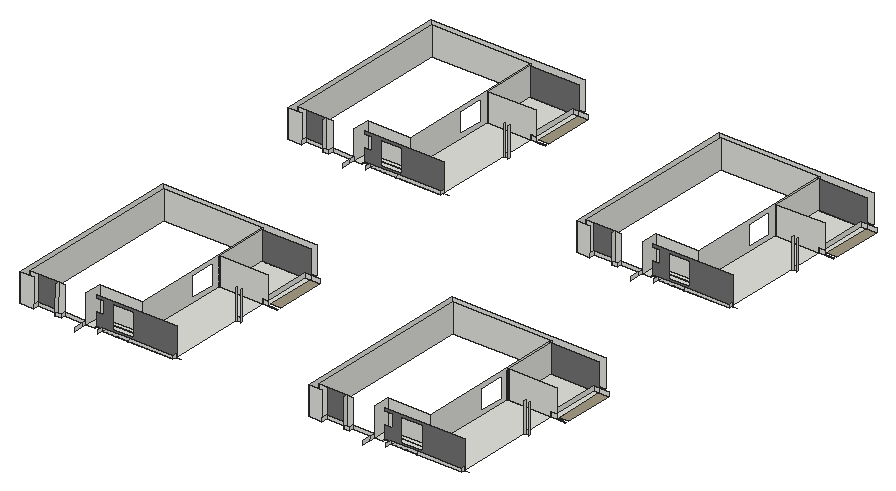
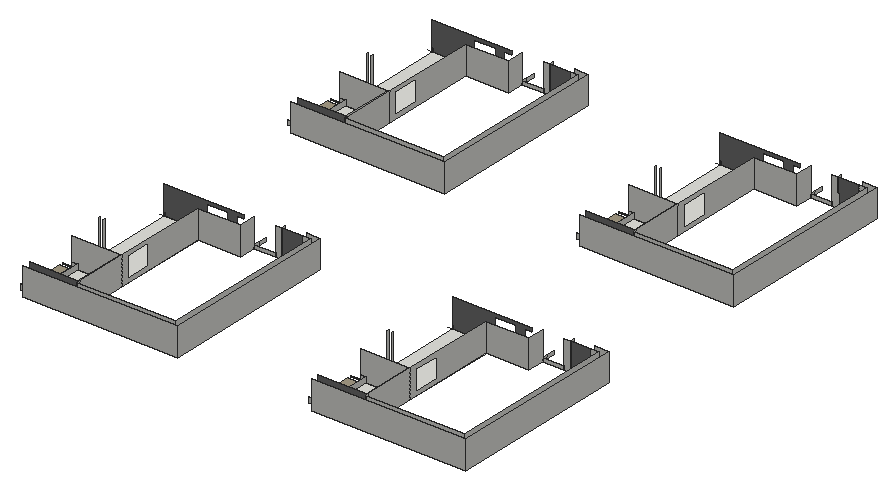
# SketchUp Ruby script. Lengths in inches.
U = 1.inch
M = Sketchup.active_model
def pt(a) = Geom::Point3d.new(a.map { |v| v * U })
def face(e, loops, mat)
  f = e.add_face(loops[0].map { |a| pt(a) })
  loops[1..].each { |l| e.add_face(l.map { |a| pt(a) }).erase! }
  f.material = f.back_material = mat if mat
  f
end
# faces: each face lists its corners as indices into pts; further lists are holes
def faces(e, pts, list, mat = nil) = list.each { |f| face(e, (f[0].is_a?(Array) ? f : [f]).map { |l| l.map { |i| pts[i] } }, mat) }
# xy, xz, yz: faces in a plane at the given z, y or x. An outline is a flat list of corners, or four numbers for a rectangle; further outlines are holes
def ring(l) = l.size == 4 ? [[l[0], l[1]], [l[2], l[1]], [l[2], l[3]], [l[0], l[3]]] : l.each_slice(2).to_a
def flat(e, list, mat, &to3) = list.each { |f| face(e, (f[0].is_a?(Array) ? f : [f]).map { |l| ring(l).map { |u, v| to3.(u, v) } }, mat) }
def xy(e, z, list, mat = nil) = flat(e, list, mat) { |x, y| [x, y, z] }
def xz(e, y, list, mat = nil) = flat(e, list, mat) { |x, z| [x, y, z] }
def yz(e, x, list, mat = nil) = flat(e, list, mat) { |y, z| [x, y, z] }
def lines(e, pts, list) = list.each { |a, b| e.add_line(pt(pts[a]), pt(pts[b])) }
# prism: a flat outline (further loops are holes) pulled along v
def prism(e, loops, v, mat = nil)
  f = face(e, loops, mat); d = Geom::Vector3d.new(v.map { |x| x * U })
  f.pushpull(f.normal.samedirection?(d) ? d.length : -d.length)
end
def box(e, o, s, mat = nil) = prism(e, [[o, [o[0] + s[0], o[1], o[2]], [o[0] + s[0], o[1] + s[1], o[2]], [o[0], o[1] + s[1], o[2]]]], [0, 0, s[2]], mat)
def at(x, y, z, deg = 0) = Geom::Transformation.translation(pt([x, y, z])) * Geom::Transformation.rotation(ORIGIN, Z_AXIS, deg.degrees)
def axes(o, x, y, z) = Geom::Transformation.new([*x, 0, *y, 0, *z, 0, *pt(o).to_a, 1])
def part(name) = M.definitions.add(name)
# library, detail: a bought-in or finely detailed component or shape, given as its bounding box
def library(name, o, s) = part(name).tap { |d| box(d.entities, o, s) }
def detail(e, o, s) = box(e.add_group.entities, o, s)
def put(e, d, t, mat = nil) = e.add_instance(d, t).tap { |i| i.material = mat if mat }
def group(e, t, mat = nil) = e.add_group.tap { |g| g.transformation = t; g.material = mat if mat }.entities
root = M.entities
M.materials.add("[Color M05]").color = [114, 114, 114]
M.materials.add("[Concrete Tile]").color = [165, 155, 133]
M.materials.add("[Granite Brown]").color = [89, 59, 61]
xy(root,1264.5625,[[653.67,1822.9375,653.67,1835.1875,557.4,1835.1875,557.4,1875.8125,704.25,1875.8125,704.25,1822.9375],[1871.86,1822.9375,1871.86,1835.1875,1775.59,1835.1875,1775.59,1875.8125,1922.4375,1875.8125,1922.4375,1822.9375],[557.4,1833.3125,653.67,1835.1875],[1775.59,1833.3125,1871.86,1835.1875],[653.67,3237.625,653.67,3249.875,557.4,3249.875,557.4,3290.5,704.25,3290.5,704.25,3237.625],
  [1871.86,3237.625,1871.86,3249.875,1775.59,3249.875,1775.59,3290.5,1922.4375,3290.5,1922.4375,3237.625],[557.4,3248,653.67,3249.875],[1775.59,3248,1871.86,3249.875]])
xy(root,1264.6875,[[653.67,1822.9375,704.25,1822.9375,704.25,1835.1875,557.4,1835.1875,557.4,1833.3125,653.67,1833.3125],[1871.86,1822.9375,1922.4375,1822.9375,1922.4375,1835.1875,1775.59,1835.1875,1775.59,1833.3125,1871.86,1833.3125],[653.67,3237.625,704.25,3237.625,704.25,3249.875,557.4,3249.875,557.4,3248,653.67,3248],[1871.86,3237.625,1922.4375,3237.625,1922.4375,3249.875,1775.59,3249.875,1775.59,3248,1871.86,3248]])
xy(root,1266,[[523.04,1822.9375,557.4,1893.6875],[704.25,1822.9375,890.875,1835.1875],[1741.23,1822.9375,1775.59,1893.6875],[1922.4375,1822.9375,2109.0625,1835.1875],[557.4,1835.1875,704.25,1875.8125],
  [704.25,1835.1875,890.875,2295.875],[1775.59,1835.1875,1922.4375,1875.8125],[1922.4375,1835.1875,2109.0625,2295.875],[557.4,1875.8125,704.25,1893.6875],[1775.59,1875.8125,1922.4375,1893.6875],
  [704.25,2295.875,710.125,2518.89],[710.125,2295.875,890.875,2518.89],[890.875,2295.875,913.875,2518.89],[1922.4375,2295.875,1928.3125,2518.89],[1928.3125,2295.875,2109.0625,2518.89],
  [2109.0625,2295.875,2132.0625,2518.89],[704.25,2518.89,890.875,2531.375],[1922.4375,2518.89,2109.0625,2531.375],[523.04,3237.625,557.4,3308.375],[704.25,3237.625,890.875,3249.875],
  [1741.23,3237.625,1775.59,3308.375],[1922.4375,3237.625,2109.0625,3249.875],[557.4,3249.875,704.25,3290.5],[704.25,3249.875,890.875,3710.5625],[1775.59,3249.875,1922.4375,3290.5],
  [1922.4375,3249.875,2109.0625,3710.5625],[557.4,3290.5,704.25,3308.375],[1775.59,3290.5,1922.4375,3308.375],[704.25,3710.5625,710.125,3933.57],[710.125,3710.5625,890.875,3933.57],
  [890.875,3710.5625,913.875,3933.57],[1922.4375,3710.5625,1928.3125,3933.57],[1928.3125,3710.5625,2109.0625,3933.57],[2109.0625,3710.5625,2132.0625,3933.57],[704.25,3933.57,890.875,3946.0625],
  [1922.4375,3933.57,2109.0625,3946.0625]])
xy(root,1266,[[913.875,2310.68,954.6875,2518.89],[2132.0625,2310.68,2172.875,2518.89],[913.875,3725.37,954.6875,3933.57],[2132.0625,3725.37,2172.875,3933.57]],"[Concrete Tile]")
xy(root,1266,[[557.4,1822.9375,557.88,1833.3125],[1775.59,1822.9375,1776.07,1833.3125],[557.4,1833.3125,557.88,1835.1875],[1775.59,1833.3125,1776.07,1835.1875],[557.4,3237.625,557.88,3248],
  [1775.59,3237.625,1776.07,3248],[557.4,3248,557.88,3249.875],[1775.59,3248,1776.07,3249.875]],"[Granite Brown]")
xz(root,1799.9375,[[262.875,1266,319.53,1386],[1481.0625,1266,1537.72,1386]])
xz(root,1806.5625,[[404.95,1266,404.95,1281.4375,405.03,1281.4375],[404.95,1266,431.33,1266,431.33,1281.4375,405.03,1281.4375],[1623.14,1266,1623.14,1281.4375,1623.22,1281.4375],[1623.14,1266,1649.52,1266,1649.52,1281.4375,1623.22,1281.4375]])
xz(root,1822.9375,[[589.79,1264.5625,653.67,1264.6875],[653.67,1264.5625,704.25,1264.6875],[1807.98,1264.5625,1871.86,1264.6875],[1871.86,1264.5625,1922.4375,1264.6875],[589.79,1264.6875,653.67,1266],
  [653.67,1264.6875,704.25,1266],[1807.98,1264.6875,1871.86,1266],[1871.86,1264.6875,1922.4375,1266],[285.875,1266,319.53,1386],[319.53,1266,404.95,1281.4375],
  [404.95,1266,405.55,1386,431.33,1386,431.33,1266],[431.33,1266,523.04,1281.4375],[589.79,1266,704.25,1278.6875],[704.25,1266,890.875,1278.6875],[1504.0625,1266,1537.72,1386],
  [1537.72,1266,1623.14,1281.4375],[1623.14,1266,1623.74,1386,1649.52,1386,1649.52,1266],[1649.52,1266,1741.23,1281.4375],[1807.98,1266,1922.4375,1278.6875],[1922.4375,1266,2109.0625,1278.6875]])
xz(root,1822.9375,[[404.95,1266,405.55,1386,319.53,1386,319.53,1281.4375,404.95,1281.4375],[1623.14,1266,1623.74,1386,1537.72,1386,1537.72,1281.4375,1623.14,1281.4375]],"[Color M05]")
xz(root,1822.9375,[[557.4,1264.5625,557.88,1266],[1775.59,1264.5625,1776.07,1266]],"[Granite Brown]")
xz(root,1833.3125,[[557.4,1264.5625,653.67,1264.6875],[1775.59,1264.5625,1871.86,1264.6875]])
xz(root,1835.1875,[[557.4,1264.6875,704.25,1266],[1775.59,1264.6875,1922.4375,1266],[890.875,1266,894.3125,1278.6875],[2109.0625,1266,2112.5,1278.6875]])
xz(root,1835.1875,[[[557.88,1266,890.875,1266,890.875,1278.6875,894.3125,1278.6875,894.3125,1386,557.88,1386,557.88,1373.32,588.66,1373.32,588.66,1321.04,557.88,1321.04],[646.53,1276.95,646.53,1277.26,625.7,1277.26,625.7,1375.08,715.63,1375.08,715.63,1276.95]],[[1776.07,1266,2109.0625,1266,2109.0625,1278.6875,2112.5,1278.6875,2112.5,1386,1776.07,1386,1776.07,1373.32,1806.84,1373.32,1806.84,1321.04,1776.07,1321.04],[1864.72,1276.95,1864.72,1277.26,1843.88,1277.26,1843.88,1375.08,1933.82,1375.08,1933.82,1276.95]]],"[Color M05]")
xz(root,1875.8125,[[557.4,1264.5625,704.25,1266],[1775.59,1264.5625,1922.4375,1266]])
xz(root,1893.6875,[[523.04,1266,704.25,1386],[1741.23,1266,1922.4375,1386]])
xz(root,2156.01,[[894.3125,1266,913.875,1283.36],[2112.5,1266,2132.0625,1283.36]])
xz(root,2295.875,[[704.25,1266,710.125,1386],[710.125,1266,710.125,1386,913.875,1386,913.875,1286.8125,890.875,1286.8125,890.875,1266],[890.875,1266,913.875,1286.8125],[913.875,1266,930.75,1267.75],[930.75,1266,954.6875,1267.75],
  [1922.4375,1266,1928.3125,1386],[1928.3125,1266,1928.3125,1386,2132.0625,1386,2132.0625,1286.8125,2109.0625,1286.8125,2109.0625,1266],[2109.0625,1266,2132.0625,1286.8125],[2132.0625,1266,2148.9375,1267.75],[2148.9375,1266,2172.875,1267.75]])
xz(root,2518.89,[[704.25,1266,710.125,1386],[890.875,1266,913.875,1286.8125],[913.875,1266,954.6875,1286.8125],[1922.4375,1266,1928.3125,1386],[2109.0625,1266,2132.0625,1286.8125],
  [2132.0625,1266,2172.875,1286.8125]])
xz(root,2518.89,[[710.125,1266,890.875,1266,890.875,1286.8125,913.875,1286.8125,913.875,1386,710.125,1386],[1928.3125,1266,2109.0625,1266,2109.0625,1286.8125,2132.0625,1286.8125,2132.0625,1386,1928.3125,1386]],"[Color M05]")
xz(root,2531.375,[[285.875,1266,704.25,1386],[1504.0625,1266,1922.4375,1386]])
xz(root,2554.375,[[262.875,1266,913.875,1386],[1481.0625,1266,2132.0625,1386]])
xz(root,3214.625,[[262.875,1266,319.53,1386],[1481.0625,1266,1537.72,1386]])
xz(root,3221.25,[[404.95,1266,404.95,1281.4375,405.03,1281.4375],[404.95,1266,431.33,1266,431.33,1281.4375,405.03,1281.4375],[1623.14,1266,1623.14,1281.4375,1623.22,1281.4375],[1623.14,1266,1649.52,1266,1649.52,1281.4375,1623.22,1281.4375]])
xz(root,3237.625,[[589.79,1264.5625,653.67,1264.6875],[653.67,1264.5625,704.25,1264.6875],[1807.98,1264.5625,1871.86,1264.6875],[1871.86,1264.5625,1922.4375,1264.6875],[589.79,1264.6875,653.67,1266],
  [653.67,1264.6875,704.25,1266],[1807.98,1264.6875,1871.86,1266],[1871.86,1264.6875,1922.4375,1266],[285.875,1266,319.53,1386],[319.53,1266,404.95,1281.4375],
  [404.95,1266,405.55,1386,431.33,1386,431.33,1266],[431.33,1266,523.04,1281.4375],[589.79,1266,704.25,1278.6875],[704.25,1266,890.875,1278.6875],[1504.0625,1266,1537.72,1386],
  [1537.72,1266,1623.14,1281.4375],[1623.14,1266,1623.74,1386,1649.52,1386,1649.52,1266],[1649.52,1266,1741.23,1281.4375],[1807.98,1266,1922.4375,1278.6875],[1922.4375,1266,2109.0625,1278.6875]])
xz(root,3237.625,[[404.95,1266,405.55,1386,319.53,1386,319.53,1281.4375,404.95,1281.4375],[1623.14,1266,1623.74,1386,1537.72,1386,1537.72,1281.4375,1623.14,1281.4375]],"[Color M05]")
xz(root,3237.625,[[557.4,1264.5625,557.88,1266],[1775.59,1264.5625,1776.07,1266]],"[Granite Brown]")
xz(root,3248,[[557.4,1264.5625,653.67,1264.6875],[1775.59,1264.5625,1871.86,1264.6875]])
xz(root,3249.875,[[557.4,1264.6875,704.25,1266],[1775.59,1264.6875,1922.4375,1266],[890.875,1266,894.3125,1278.6875],[2109.0625,1266,2112.5,1278.6875]])
xz(root,3249.875,[[[557.88,1266,890.875,1266,890.875,1278.6875,894.3125,1278.6875,894.3125,1386,557.88,1386,557.88,1373.32,588.66,1373.32,588.66,1321.04,557.88,1321.04],[646.53,1276.95,646.53,1277.26,625.7,1277.26,625.7,1375.08,715.63,1375.08,715.63,1276.95]],[[1776.07,1266,2109.0625,1266,2109.0625,1278.6875,2112.5,1278.6875,2112.5,1386,1776.07,1386,1776.07,1373.32,1806.84,1373.32,1806.84,1321.04,1776.07,1321.04],[1864.72,1276.95,1864.72,1277.26,1843.88,1277.26,1843.88,1375.08,1933.82,1375.08,1933.82,1276.95]]],"[Color M05]")
xz(root,3290.5,[[557.4,1264.5625,704.25,1266],[1775.59,1264.5625,1922.4375,1266]])
xz(root,3308.375,[[523.04,1266,704.25,1386],[1741.23,1266,1922.4375,1386]])
xz(root,3570.7,[[894.3125,1266,913.875,1283.36],[2112.5,1266,2132.0625,1283.36]])
xz(root,3710.5625,[[704.25,1266,710.125,1386],[710.125,1266,710.125,1386,913.875,1386,913.875,1286.8125,890.875,1286.8125,890.875,1266],[890.875,1266,913.875,1286.8125],[913.875,1266,930.75,1267.75],[930.75,1266,954.6875,1267.75],
  [1922.4375,1266,1928.3125,1386],[1928.3125,1266,1928.3125,1386,2132.0625,1386,2132.0625,1286.8125,2109.0625,1286.8125,2109.0625,1266],[2109.0625,1266,2132.0625,1286.8125],[2132.0625,1266,2148.9375,1267.75],[2148.9375,1266,2172.875,1267.75]])
xz(root,3933.57,[[704.25,1266,710.125,1386],[890.875,1266,913.875,1286.8125],[913.875,1266,954.6875,1286.8125],[1922.4375,1266,1928.3125,1386],[2109.0625,1266,2132.0625,1286.8125],
  [2132.0625,1266,2172.875,1286.8125]])
xz(root,3933.57,[[710.125,1266,890.875,1266,890.875,1286.8125,913.875,1286.8125,913.875,1386,710.125,1386],[1928.3125,1266,2109.0625,1266,2109.0625,1286.8125,2132.0625,1286.8125,2132.0625,1386,1928.3125,1386]],"[Color M05]")
xz(root,3946.0625,[[285.875,1266,704.25,1386],[1504.0625,1266,1922.4375,1386]])
xz(root,3969.0625,[[262.875,1266,913.875,1386],[1481.0625,1266,2132.0625,1386]])
yz(root,262.875,[[1799.9375,1266,2554.375,1386],[3214.625,1266,3969.0625,1386]])
yz(root,285.875,[[1822.9375,1266,2531.375,1386],[3237.625,1266,3946.0625,1386]])
yz(root,319.53,[[1799.9375,1266,1822.9375,1281.4375],[3214.625,1266,3237.625,1281.4375]])
yz(root,404.95,[[1806.5625,1266,1822.9375,1281.4375],[3221.25,1266,3237.625,1281.4375]])
yz(root,431.33,[[1806.5625,1266,1822.9375,1281.4375],[3221.25,1266,3237.625,1281.4375]])
yz(root,523.04,[[1763.25,1266,1799.9375,1281.4375],[1799.9375,1266,1822.9375,1281.4375],[1822.9375,1266,1893.6875,1386],[3177.9375,1266,3214.625,1281.4375],[3214.625,1266,3237.625,1281.4375],
  [3237.625,1266,3308.375,1386]])
yz(root,557.4,[[1822.9375,1264.5625,1833.3125,1266],[1833.3125,1264.5625,1833.3125,1264.6875,1835.1875,1264.6875,1835.1875,1266,1875.8125,1266,1875.8125,1264.5625],[3237.625,1264.5625,3248,1266],[3248,1264.5625,3248,1264.6875,3249.875,1264.6875,3249.875,1266,3290.5,1266,3290.5,1264.5625],[1833.3125,1264.6875,1835.1875,1266],
  [3248,1264.6875,3249.875,1266]])
yz(root,589.79,[[1799.9375,1266,1822.9375,1278.6875],[3214.625,1266,3237.625,1278.6875]])
yz(root,653.67,[[1822.9375,1264.5625,1833.3125,1264.6875],[3237.625,1264.5625,3248,1264.6875],[1822.9375,1264.6875,1833.3125,1266],[3237.625,1264.6875,3248,1266]])
yz(root,704.25,[[1822.9375,1264.5625,1875.8125,1264.5625,1875.8125,1266,1835.1875,1266,1835.1875,1264.6875,1822.9375,1264.6875],[3237.625,1264.5625,3290.5,1264.5625,3290.5,1266,3249.875,1266,3249.875,1264.6875,3237.625,1264.6875],[1822.9375,1264.6875,1835.1875,1266],[3237.625,1264.6875,3249.875,1266],[[1893.6875,1266,2295.875,1386],[2156.01,1283.36,2266.33,1369.04]],
  [2295.875,1266,2518.89,1386],[2518.89,1266,2531.375,1386],[[3308.375,1266,3710.5625,1386],[3570.7,1283.36,3681.01,1369.04]],[3710.5625,1266,3933.57,1386],[3933.57,1266,3946.0625,1386]])
yz(root,710.125,[[2295.875,1266,2518.89,1386],[3710.5625,1266,3933.57,1386]])
yz(root,890.875,[[1822.9375,1266,1835.1875,1278.6875],[2295.875,1266,2518.89,1286.8125],[3237.625,1266,3249.875,1278.6875],[3710.5625,1266,3933.57,1286.8125]])
yz(root,894.3125,[[2148.83,1266,2156.01,1392],[3563.51,1266,3570.7,1392]])
yz(root,913.875,[[2148.83,1266,2156.01,1392],[3563.51,1266,3570.7,1392]])
yz(root,1481.0625,[[1799.9375,1266,2554.375,1386],[3214.625,1266,3969.0625,1386]])
yz(root,1504.0625,[[1822.9375,1266,2531.375,1386],[3237.625,1266,3946.0625,1386]])
yz(root,1537.72,[[1799.9375,1266,1822.9375,1281.4375],[3214.625,1266,3237.625,1281.4375]])
yz(root,1623.14,[[1806.5625,1266,1822.9375,1281.4375],[3221.25,1266,3237.625,1281.4375]])
yz(root,1649.52,[[1806.5625,1266,1822.9375,1281.4375],[3221.25,1266,3237.625,1281.4375]])
yz(root,1741.23,[[1763.25,1266,1799.9375,1281.4375],[1799.9375,1266,1822.9375,1281.4375],[1822.9375,1266,1893.6875,1386],[3177.9375,1266,3214.625,1281.4375],[3214.625,1266,3237.625,1281.4375],
  [3237.625,1266,3308.375,1386]])
yz(root,1775.59,[[1822.9375,1264.5625,1833.3125,1266],[1833.3125,1264.5625,1833.3125,1264.6875,1835.1875,1264.6875,1835.1875,1266,1875.8125,1266,1875.8125,1264.5625],[3237.625,1264.5625,3248,1266],[3248,1264.5625,3248,1264.6875,3249.875,1264.6875,3249.875,1266,3290.5,1266,3290.5,1264.5625],[1833.3125,1264.6875,1835.1875,1266],
  [3248,1264.6875,3249.875,1266]])
yz(root,1807.98,[[1799.9375,1266,1822.9375,1278.6875],[3214.625,1266,3237.625,1278.6875]])
yz(root,1871.86,[[1822.9375,1264.5625,1833.3125,1264.6875],[3237.625,1264.5625,3248,1264.6875],[1822.9375,1264.6875,1833.3125,1266],[3237.625,1264.6875,3248,1266]])
yz(root,1922.4375,[[1822.9375,1264.5625,1875.8125,1264.5625,1875.8125,1266,1835.1875,1266,1835.1875,1264.6875,1822.9375,1264.6875],[3237.625,1264.5625,3290.5,1264.5625,3290.5,1266,3249.875,1266,3249.875,1264.6875,3237.625,1264.6875],[1822.9375,1264.6875,1835.1875,1266],[3237.625,1264.6875,3249.875,1266],[[1893.6875,1266,2295.875,1386],[2156.01,1283.36,2266.33,1369.04]],
  [2295.875,1266,2518.89,1386],[2518.89,1266,2531.375,1386],[[3308.375,1266,3710.5625,1386],[3570.7,1283.36,3681.01,1369.04]],[3710.5625,1266,3933.57,1386],[3933.57,1266,3946.0625,1386]])
yz(root,1928.3125,[[2295.875,1266,2518.89,1386],[3710.5625,1266,3933.57,1386]])
yz(root,2109.0625,[[1822.9375,1266,1835.1875,1278.6875],[2295.875,1266,2518.89,1286.8125],[3237.625,1266,3249.875,1278.6875],[3710.5625,1266,3933.57,1286.8125]])
yz(root,2112.5,[[2148.83,1266,2156.01,1392],[3563.51,1266,3570.7,1392]])
yz(root,2132.0625,[[2148.83,1266,2156.01,1392],[3563.51,1266,3570.7,1392]])
p = [[404.95,1822.9375,1266],[404.95,1806.5625,1266],[405.03,1806.5625,1281.4375],[405.55,1806.5625,1386],[405.55,1822.9375,1386],[1623.14,1822.9375,1266],
  [1623.14,1806.5625,1266],[1623.22,1806.5625,1281.4375],[1623.74,1806.5625,1386],[1623.74,1822.9375,1386],[404.95,3237.625,1266],[404.95,3221.25,1266],
  [405.03,3221.25,1281.4375],[405.55,3221.25,1386],[405.55,3237.625,1386],[1623.14,3237.625,1266],[1623.14,3221.25,1266],[1623.22,3221.25,1281.4375],
  [1623.74,3221.25,1386],[1623.74,3237.625,1386],[2112.5,1835.1875,1266],[2132.0625,1835.1875,1266],[894.3125,1835.1875,1266],[913.875,1835.1875,1266],
  [2112.5,3249.875,1266],[2132.0625,3249.875,1266],[894.3125,3249.875,1266],[913.875,3249.875,1266]]
faces(root,p,[[0,1,2,3,4],[5,6,7,8,9],[10,11,12,13,14],[15,16,17,18,19]])
lines(root,p,[[20,21],[22,23],[24,25],[26,27]])
